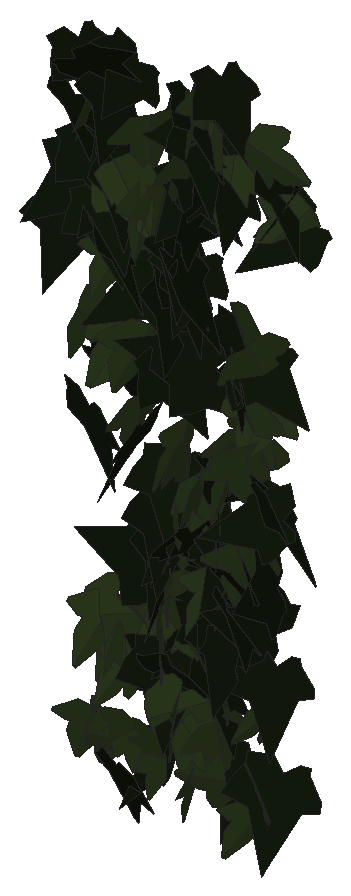
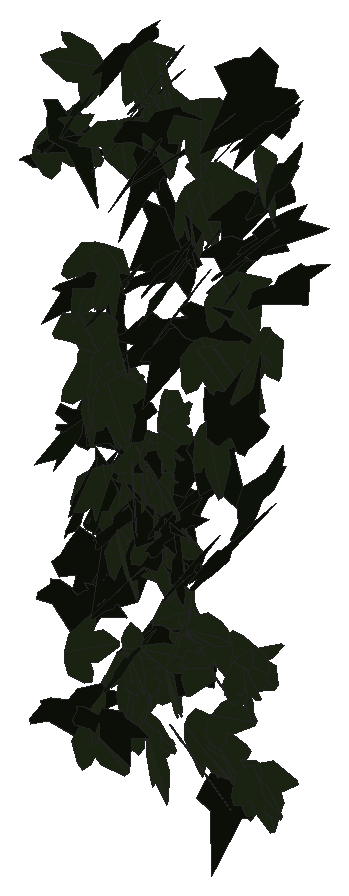
# SketchUp Ruby script. Lengths in inches.
U = 1.inch
M = Sketchup.active_model
def pt(a) = Geom::Point3d.new(a.map { |v| v * U })
def face(e, loops, mat)
  f = e.add_face(loops[0].map { |a| pt(a) })
  loops[1..].each { |l| e.add_face(l.map { |a| pt(a) }).erase! }
  f.material = f.back_material = mat if mat
  f
end
# faces: each face lists its corners as indices into pts; further lists are holes
def faces(e, pts, list, mat = nil) = list.each { |f| face(e, (f[0].is_a?(Array) ? f : [f]).map { |l| l.map { |i| pts[i] } }, mat) }
# xy, xz, yz: faces in a plane at the given z, y or x. An outline is a flat list of corners, or four numbers for a rectangle; further outlines are holes
def ring(l) = l.size == 4 ? [[l[0], l[1]], [l[2], l[1]], [l[2], l[3]], [l[0], l[3]]] : l.each_slice(2).to_a
def flat(e, list, mat, &to3) = list.each { |f| face(e, (f[0].is_a?(Array) ? f : [f]).map { |l| ring(l).map { |u, v| to3.(u, v) } }, mat) }
def xy(e, z, list, mat = nil) = flat(e, list, mat) { |x, y| [x, y, z] }
def xz(e, y, list, mat = nil) = flat(e, list, mat) { |x, z| [x, y, z] }
def yz(e, x, list, mat = nil) = flat(e, list, mat) { |y, z| [x, y, z] }
def lines(e, pts, list) = list.each { |a, b| e.add_line(pt(pts[a]), pt(pts[b])) }
# prism: a flat outline (further loops are holes) pulled along v
def prism(e, loops, v, mat = nil)
  f = face(e, loops, mat); d = Geom::Vector3d.new(v.map { |x| x * U })
  f.pushpull(f.normal.samedirection?(d) ? d.length : -d.length)
end
def box(e, o, s, mat = nil) = prism(e, [[o, [o[0] + s[0], o[1], o[2]], [o[0] + s[0], o[1] + s[1], o[2]], [o[0], o[1] + s[1], o[2]]]], [0, 0, s[2]], mat)
def at(x, y, z, deg = 0) = Geom::Transformation.translation(pt([x, y, z])) * Geom::Transformation.rotation(ORIGIN, Z_AXIS, deg.degrees)
def axes(o, x, y, z) = Geom::Transformation.new([*x, 0, *y, 0, *z, 0, *pt(o).to_a, 1])
def part(name) = M.definitions.add(name)
# library, detail: a bought-in or finely detailed component or shape, given as its bounding box
def library(name, o, s) = part(name).tap { |d| box(d.entities, o, s) }
def detail(e, o, s) = box(e.add_group.entities, o, s)
def put(e, d, t, mat = nil) = e.add_instance(d, t).tap { |i| i.material = mat if mat }
def group(e, t, mat = nil) = e.add_group.tap { |g| g.transformation = t; g.material = mat if mat }.entities
root = M.entities
M.materials.add("efeu1").color = [18, 25, 13]
M.materials.add("efeu2").color = [43, 57, 29]
c1 = part("ivyleaf_10")
p = [[0,0.5,-0.03],[-0.0625,2.02,-0.43],[-0.19,2.01,-0.46],[-0.54,1.05,-0.29],[-0.52,0.625,-0.18],[-0.83,0.76,-0.28],
  [-1.16,0.64,-0.33],[-1.15,0.33,-0.24],[-0.77,-0.39,0.02],[-0.3,-0.51,0.16],[0.04,-0.48,0.23],[-0.02,2.01,-0.4375],
  [-0.06,2.01,-0.43],[0.04,-0.49,0.23],[0.67,-0.49,0.14],[1.38,0.36,-0.2],[1.375,0.51,-0.24],[0.81,0.65,-0.19],
  [0.62,0.59,-0.15],[0.6,1.09,-0.28],[0.5,1.23,-0.31]]
faces(c1.entities,p,[[0,1,2,3,4,5,6,7,8,9,10],[11,12,0,13,14,15,16,17,18,19,20]],"efeu2")
c2 = part("ivyleaf_9")
p = [[1.54,2.16,1.25],[1.36,2.04,1.19],[-0.21,0.99,0.68],[-0.71,1.11,0.82],[-0.85,0.86,0.67],[-0.8,0.17,0.21],
  [-0.9,-0.01,0.1],[-0.67,-0.16,-0.02],[-0.08,-0.08,-0.05],[-0.03,-0.6,-0.4],[0.65,-0.88,-0.66],[0.83,-0.6,-0.49],
  [1.29,-0.42,-0.43],[1.8125,-0.07,-0.26],[1.21,0.44,0.15]]
faces(c2.entities,p,[[0,1,2,3,4,5,6,7,8,9,10,11,12,13,14]],"efeu1")
put(root,c1,axes([532.02,132.86,205.625],[0.54701,-0.58497,-0.26484],[-0.14325,0.22798,-0.79941],[0.62595,0.56337,0.04849]))
put(root,c1,axes([531.9,133,204.33],[-0.00085,-0.92422,-0.0039],[-0.00106,0.0039,-0.92422],[0.92423,-0.00084,-0.00107]))
put(root,c2,axes([532,133.3,204.76],[0.15563,-0.81555,0.1224],[0.07979,-0.10908,-0.82829],[0.82082,0.16524,0.05731]))
put(root,c2,axes([530.08,133.48,190.96],[0.09192,-0.89699,-0.19736],[0.02627,-0.1957,0.90167],[-0.91807,-0.09541,0.00604]))
put(root,c1,axes([530.97,133.13,191.32],[-0.41441,0.49964,-0.41549],[0.14606,-0.40856,-0.63699],[-0.63319,-0.42125,0.125]))
put(root,c1,axes([532.94,133.45,195],[0.0785,-0.55553,0.59073],[0.29926,-0.53176,-0.53984],[0.75368,0.269,0.15282]))
put(root,c2,axes([533.09,133.53,190.52],[0.17952,-0.61811,0.57461],[0.20391,-0.5383,-0.64274],[0.81894,0.26953,0.03408]))
put(root,c2,axes([528.87,133.62,204.78],[-0.04827,-0.74776,0.44056],[0.06981,-0.44315,-0.74452],[0.86508,-0.00596,0.08467]))
put(root,c1,axes([531.32,132.64,187.23],[0.20508,0.09961,-0.82729],[0.75248,0.3438,0.22793],[0.3579,-0.77991,-0.00518]))
put(root,c1,axes([529.61,132.87,202.91],[0.64103,0.38188,0.45288],[0.39221,0.2265,-0.74614],[-0.44397,0.75147,-0.00526]))
put(root,c2,axes([527.93,133.67,202.14],[-0.41899,-0.53929,0.51799],[-0.29131,-0.42913,-0.68241],[0.68868,-0.50962,0.02648]))
put(root,c1,axes([531.3125,133.3,187.21],[0.37585,-0.57183,0.34634],[0.24164,-0.25427,-0.68203],[0.62334,0.44336,0.05555]))
put(root,c2,axes([531.07,133.25,188.54],[-0.5829,-0.53277,-0.42244],[0.3041,0.29339,-0.78963],[0.60813,-0.65738,-0.01005]))
put(root,c2,axes([534.25,133.73,191.54],[-0.06538,-0.32194,0.83628],[-0.19736,-0.81274,-0.32831],[0.8741,-0.20758,-0.01158]))
put(root,c2,axes([531.7,133.6875,202.84],[-0.36375,-0.5854,0.46056],[0.00311,-0.51374,-0.65053],[0.74485,-0.28373,0.22764]))
put(root,c2,axes([533.47,133.58,191.86],[0.08581,-0.37368,0.77978],[0.24054,-0.74237,-0.38222],[0.83056,0.25361,0.03013]))
put(root,c2,axes([530.9375,133.47,191.24],[-0.23283,0.02472,-0.74149],[0.60895,-0.43756,-0.20579],[-0.42379,-0.64231,0.11166]))
put(root,c1,axes([530.11,133.38,202.23],[0.02057,-0.74127,0.36329],[0.24871,-0.34095,-0.70977],[0.78715,0.1271,0.21477]))
put(root,c1,axes([533.9,133.36,184.67],[-0.31046,-0.5235,0.43837],[-0.19234,-0.39501,-0.60793],[0.65515,-0.36404,0.02926]))
put(root,c2,axes([527.47,133.59,200.8125],[-0.30848,-0.78065,0.13568],[-0.03516,-0.13197,-0.83924],[0.79157,-0.31008,0.0156]))
put(root,c2,axes([531.32,133.14,200.76],[-0.21208,-0.05665,-0.91189],[0.85014,0.33069,-0.21826],[0.33469,-0.87588,-0.02342]))
put(root,c1,axes([530.51,133.07,204.72],[-0.445,-0.70945,-0.04313],[0.02158,0.03738,-0.83747],[0.71044,-0.44552,-0.00159]))
put(root,c2,axes([530.61,132.91,188.07],[0.30461,0.20191,-0.67109],[0.53531,0.40522,0.3649],[0.45229,-0.61558,0.02009]))
put(root,c2,axes([530.75,133.58,192.82],[-0.0974,-0.86981,0.11578],[-0.01013,-0.11537,-0.87524],[0.87742,-0.09789,0.00275]))
put(root,c1,axes([532.76,133.09,185.51],[-0.19611,0.02326,0.77628],[-0.77293,-0.08384,-0.19275],[0.07566,-0.79626,0.04297]))
put(root,c1,axes([532.8,133.05,187.0625],[-0.32522,-0.69186,-0.17785],[0.09706,0.1508,-0.76413],[0.70772,-0.33861,0.02307]))
put(root,c2,axes([528.99,133.6,202.4],[0.15948,-0.75012,0.28949],[0.07702,-0.27952,-0.76671],[0.80034,0.17637,0.0161]))
put(root,c2,axes([531.75,133.24,192.55],[-0.19968,0.63241,-0.49087],[0.06118,-0.49237,-0.65924],[-0.79822,-0.19594,0.07227]))
put(root,c2,axes([534.65,133.39,193.92],[-0.6743,0.00539,0.4409],[-0.44088,0.00467,-0.67432],[-0.00707,-0.80564,-0.00096]))
put(root,c2,axes([533.64,132.86,198.11],[0.13195,0.04339,-0.81934],[-0.81811,0.07003,-0.12804],[0.06236,0.82693,0.05383]))
put(root,c2,axes([532.57,132.85,190.33],[-0.16425,0.3405,0.69057],[-0.49762,0.49188,-0.36089],[-0.58755,-0.51178,0.1126]))
put(root,c2,axes([532.75,133.7,189.57],[-0.12607,-0.79959,0.20005],[0.00302,-0.20282,-0.80877],[0.82423,-0.12155,0.03356]))
put(root,c1,axes([532.54,133.59,191.13],[-0.36468,-0.56042,0.50547],[-0.09343,-0.52355,-0.64787],[0.7489,-0.33821,0.16532]))
put(root,c1,axes([530.75,132.93,185.55],[0.25194,-0.13166,-0.83357],[-0.69673,0.45841,-0.28299],[0.47618,0.74039,0.02697]))
put(root,c1,axes([531.64,133,195.34],[0.16512,-0.75649,-0.37081],[0.00109,0.37806,-0.77079],[0.84249,0.14778,0.07367]))
put(root,c2,axes([528.83,133.46,200.52],[0.44167,-0.6628,0.18007],[0.09977,-0.14991,-0.79647],[0.67954,0.4528,-0.0001]))
put(root,c1,axes([534.08,132.98,198.99],[-0.41179,-0.65559,-0.37988],[0.205,0.31983,-0.77419],[0.72944,-0.45999,0.00312]))
put(root,c2,axes([528.39,132.69,206.13],[0.73102,0.45301,0.21296],[0.16798,0.13306,-0.85968],[-0.47154,0.74969,0.0239]))
put(root,c1,axes([532.04,132.87,186.73],[0.06735,0.69163,0.36124],[0.04577,0.35846,-0.69483],[-0.77894,0.08086,-0.00959]))
put(root,c1,axes([529.9,133.52,197.82],[-0.42474,-0.67976,0.39362],[-0.15361,-0.36696,-0.79947],[0.77033,-0.44798,0.05761]))
put(root,c1,axes([534.11,133.32,205.1],[-0.23144,0.00481,-0.83159],[0.79681,-0.24578,-0.22318],[-0.23802,-0.82746,0.06145]))
put(root,c1,axes([533.61,133.3,192.45],[-0.64016,-0.52196,0.17914],[-0.13322,-0.12008,-0.82593],[0.53552,-0.65381,0.00868]))
put(root,c2,axes([532.02,133.79,197.51],[-0.31771,-0.72583,-0.52401],[-0.15763,-0.50199,0.79089],[-0.88123,0.35147,0.04745]))
put(root,c1,axes([533.76,133.18,195.65],[-0.60068,-0.74217,-0.1277],[0.08212,0.09782,-0.95479],[0.74858,-0.60627,0.00227]))
put(root,c2,axes([528.72,133.4375,201.62],[-0.17194,-0.7198,-0.35832],[0.18994,0.31969,-0.73334],[0.7813,-0.23612,0.09942]))
put(root,c1,axes([533.62,133.58,185.35],[-0.03842,-0.19654,0.74734],[0.70333,-0.31884,-0.0477],[0.3201,0.677,0.1945]))
put(root,c1,axes([528.41,133.82,188.77],[-0.34827,-0.45388,0.61207],[0.12453,-0.69782,-0.44662],[0.75175,-0.09469,0.35754]))
put(root,c1,axes([532.24,133.375,204.76],[0.76263,-0.35159,-0.01271],[-0.00688,0.01542,-0.8397],[0.35175,0.76258,0.01112]))
put(root,c2,axes([531.06,133.14,197.77],[0.15772,-0.65442,-0.58031],[-0.1554,0.55932,-0.67298],[0.86074,0.22089,-0.01517]))
put(root,c2,axes([531.06,133.5625,194.3],[-0.38912,-0.69537,-0.25303],[0.12177,0.22181,-0.79684],[0.72989,-0.40773,-0.00196]))
put(root,c1,axes([529.4,133.42,197.83],[0.82236,0.1954,-0.41509],[-0.4076,-0.07991,-0.84513],[-0.21059,0.91771,0.01479]))
put(root,c1,axes([531.02,133.78,195.02],[0.11228,-0.51871,0.57243],[0.1497,-0.55287,-0.53035],[0.75784,0.18606,0.01996]))
put(root,c2,axes([530.67,133.87,198.95],[0.07447,-0.7399,0.40506],[0.03071,-0.40398,-0.74359],[0.84296,0.08008,-0.00869]))
put(root,c2,axes([532.3,132.72,202.99],[0.13563,-0.12002,-0.95271],[-0.68535,0.66184,-0.18094],[0.67258,0.6986,0.00775]))
put(root,c2,axes([531.0625,133.93,192.04],[-0.20968,-0.564,0.47955],[-0.17641,-0.44599,-0.60167],[0.71899,-0.27391,-0.00777]))
put(root,c2,axes([532.69,133.88,203.43],[-0.00028,-0.75848,0.35794],[0.06685,-0.35682,-0.75606],[0.83603,0.02828,0.06058]))
put(root,c1,axes([533.77,133.28,196.86],[-0.75604,0.05552,-0.23432],[0.22904,-0.07256,-0.75621],[-0.07434,-0.78819,0.05311]))
put(root,c1,axes([530.57,133.6,189.42],[-0.16834,0.66822,-0.51384],[0.13799,-0.49507,-0.68902],[-0.83157,-0.21743,-0.01032]))
put(root,c2,axes([529.85,133.46,195.01],[-0.44426,0.58846,-0.47549],[0.27568,-0.38758,-0.73724],[-0.70454,-0.52272,0.01135]))
put(root,c2,axes([531.55,133.53,205.7],[0.41351,-0.7399,-0.03157],[-0.01315,0.02882,-0.8476],[0.74046,0.41371,0.00258]))
put(root,c2,axes([533.24,133.24,194.93],[0.23175,0.36283,-0.66877],[-0.56834,-0.38224,-0.40433],[-0.50585,0.59569,0.14789]))
put(root,c1,axes([528.36,132.92,198.3],[0.02079,-0.59617,-0.63833],[0.226,0.62044,-0.5721],[0.84369,-0.15151,0.16898]))
put(root,c1,axes([531.54,133.36,191.41],[-0.72603,-0.29018,0.16338],[-0.14034,-0.08877,-0.78131],[0.302,-0.73887,0.02971]))
put(root,c1,axes([532.125,133.65,205.95],[-0.06375,-0.80108,0.27625],[0.12177,-0.28281,-0.79202],[0.83858,-0.01983,0.13601]))
put(root,c1,axes([534.04,133.48,197.23],[0.81915,0.21802,-0.21675],[-0.21124,-0.049,-0.84764],[-0.22336,0.84592,0.00676]))
put(root,c1,axes([530.45,133.58,202.32],[0.0232,-0.81164,0.15371],[0.10795,-0.14947,-0.80556],[0.81898,0.0427,0.10183]))
put(root,c2,axes([533.89,133.27,198.55],[0.18121,-0.55981,-0.54317],[0.15185,0.57229,-0.53916],[0.76509,0.01901,0.23566]))
put(root,c2,axes([529.33,133.13,184.62],[0.68316,0.08931,-0.52708],[-0.52709,-0.03019,-0.68829],[-0.08921,0.86232,0.03049]))
put(root,c1,axes([529.51,133.32,185.69],[0.48392,-0.11141,-0.56654],[-0.5104,0.26307,-0.48769],[0.26996,0.69709,0.0935]))
put(root,c2,axes([532.86,133.07,193.57],[0.07781,-0.05125,-0.83119],[-0.79768,0.23516,-0.08918],[0.23916,0.80102,-0.027]))
put(root,c1,axes([528.81,133.54,188.4],[0.66233,-0.35838,-0.04558],[-0.04121,0.01961,-0.75306],[0.35891,0.6636,-0.00236]))
put(root,c2,axes([530.67,133.61,185.625],[-0.76016,0.22241,-0.20945],[0.20063,-0.06015,-0.79203],[-0.2304,-0.78619,0.00135]))
put(root,c1,axes([530.6,133.44,189.63],[0.39485,-0.03108,0.66099],[0.65552,0.12348,-0.38577],[-0.09036,0.75997,0.08971]))
put(root,c2,axes([534.34,133.87,185.74],[-0.41247,-0.80289,-0.14445],[0.06696,0.12799,-0.90264],[0.81302,-0.41787,0.00106]))
put(root,c1,axes([528.91,133.85,200.14],[-0.37708,-0.58511,0.42867],[-0.06931,-0.45186,-0.67774],[0.72202,-0.34896,0.15882]))
put(root,c2,axes([532.61,134.1,191.91],[-0.18755,-0.67235,0.37039],[-0.11821,-0.35144,-0.69781],[0.75847,-0.22103,-0.01717]))
put(root,c1,axes([534.74,134.05,202.9],[-0.34039,-0.35279,0.70404],[-0.14855,-0.72446,-0.43484],[0.77334,-0.29444,0.22636]))
put(root,c2,axes([533.9,134.02,189.93],[-0.03255,-0.02825,0.82963],[-0.68279,-0.47128,-0.04284],[0.47211,-0.68354,-0.00475]))
put(root,c2,axes([530.77,133.1875,188.59],[-0.37805,0.45583,0.49738],[-0.3044,0.39357,-0.59206],[-0.60209,-0.4852,-0.01297]))
put(root,c1,axes([531.59,133.67,185.04],[0.25174,-0.71675,0.0603],[0.01898,-0.05724,-0.75968],[0.71904,0.25245,-0.00106]))
put(root,c2,axes([532.82,134.07,198.625],[0.0468,-0.72136,0.40497],[0.11941,-0.39548,-0.71826],[0.8186,0.09893,0.08162]))
put(root,c2,axes([532.0625,134,187.98],[0.26419,-0.79338,0.35827],[0.15075,-0.32705,-0.83541],[0.85736,0.30198,0.03649]))
put(root,c2,axes([527.1875,134.02,203.99],[0.16824,-0.68104,0.48598],[0.25372,-0.43084,-0.69159],[0.79726,0.28082,0.11754]))
put(root,c2,axes([534.25,133.74,189.05],[-0.53997,-0.48823,-0.41615],[0.29295,0.29625,-0.72769],[0.57073,-0.61399,-0.0202]))
put(root,c2,axes([531.7,133.37,203.56],[0.50849,-0.54488,-0.44211],[-0.22051,0.39424,-0.73951],[0.66613,0.54644,0.09268]))
put(root,c2,axes([530.25,134.14,191.1],[-0.03594,-0.71087,0.4263],[0.00757,-0.42697,-0.71134],[0.82886,-0.02692,0.02498]))
put(root,c1,axes([533.84,134.16,187.5625],[0.01218,-0.16551,0.77293],[0.09618,-0.76697,-0.16575],[0.78458,0.09659,0.00832]))
put(root,c1,axes([532.62,133.72,191.08],[0.38821,-0.70909,0.03542],[0.0099,-0.03496,-0.80837],[0.70991,0.38825,-0.00809]))
put(root,c2,axes([532.48,133.68,206.46],[0.21299,-0.76786,-0.27667],[-0.05202,0.27259,-0.79656],[0.81453,0.21819,0.02147]))
put(root,c2,axes([532.49,133.25,191.53],[0.88769,0.19627,-0.27277],[-0.26574,-0.06161,-0.90912],[-0.20569,0.9266,-0.00267]))
put(root,c2,axes([528.19,133.64,203.3125],[0.0455,-0.81472,-0.45597],[0.00049,0.45653,-0.81568],[0.93364,0.03946,0.02265]))
put(root,c1,axes([527.88,133.75,204.29],[0.40436,-0.75752,0.05912],[0.02649,-0.05288,-0.85869],[0.75936,0.40523,-0.00153]))
put(root,c1,axes([528.9,134.14,187.22],[-0.23652,-0.29597,0.6492],[0.11012,-0.69089,-0.27485],[0.70493,0.00862,0.26076]))
put(root,c1,axes([528,133.68,185.51],[-0.61577,-0.33553,0.25023],[-0.20936,-0.13854,-0.70096],[0.36244,-0.65007,0.02023]))
put(root,c1,axes([531.41,133.32,193.14],[-0.17287,0.69239,0.3044],[-0.19944,0.25946,-0.70345],[-0.72958,-0.23499,0.12018]))
put(root,c2,axes([531.3,133.21,201.11],[-0.06232,0.12848,0.87859],[-0.43987,0.76062,-0.14243],[-0.77133,-0.44414,0.01023]))
put(root,c2,axes([534.09,133.75,194.24],[0.60191,-0.66537,-0.00201],[-0.0013,0.00154,-0.89722],[0.66537,0.60191,0.00007]))
put(root,c2,axes([534.12,134.01,203.8],[0.29613,-0.74041,0.23584],[0.11727,-0.20691,-0.79684],[0.76816,0.31702,0.03073]))
put(root,c1,axes([531.94,133.37,194.13],[0.13591,-0.68549,-0.46636],[-0.03339,0.46768,-0.69716],[0.82842,0.13131,0.04841]))
put(root,c1,axes([528.52,133.53,185.125],[-0.15938,0.05236,0.7381],[-0.73942,0.01748,-0.16091],[-0.02818,-0.75491,0.04747]))
put(root,c1,axes([532.75,133.72,203.78],[0.62588,0.55172,-0.09423],[-0.07828,-0.05367,-0.83426],[-0.55421,0.63065,0.01143]))
put(root,c1,axes([533.2,133.88,195.79],[0.02519,-0.77462,0.1506],[-0.01404,-0.15109,-0.77481],[0.789,0.02204,-0.01859]))
put(root,c1,axes([532.76,133.28,187.63],[0.17921,-0.14057,-0.81291],[-0.51976,0.62677,-0.22297],[0.64065,0.54781,0.04651]))
put(root,c1,axes([532.89,133.86,195.59],[-0.14946,-0.75542,0.15525],[-0.01017,-0.1562,-0.7698],[0.77114,-0.14847,0.01994]))
put(root,c2,axes([531.43,134.09,204.63],[-0.43645,-0.74024,-0.11235],[0.05193,0.09981,-0.85931],[0.74692,-0.43949,-0.00591]))
put(root,c1,axes([528.34,133.63,188.79],[0.24505,-0.08512,-0.88949],[0.89094,-0.04729,0.24997],[-0.06836,-0.92142,0.06934]))
put(root,c2,axes([534.88,134.3,202.625],[-0.57951,-0.41741,0.38754],[-0.22401,-0.34129,-0.70256],[0.52368,-0.6079,0.12833]))
put(root,c1,axes([531.87,133.6,193.97],[-0.38654,-0.61967,-0.34452],[0.32702,0.19234,-0.71286],[0.62908,-0.48074,0.15888]))
put(root,c2,axes([533.18,134.01,185.71],[-0.6546,-0.35747,-0.23831],[0.20488,0.12202,-0.7458],[0.37763,-0.68586,-0.00847]))
put(root,c2,axes([530.82,134.125,199.71],[0.27974,-0.74988,0.2179],[0.07008,-0.20642,-0.80033],[0.77775,0.28831,-0.00626]))
put(root,c2,axes([528.71,133.95,196],[0.661,-0.36637,0.42115],[-0.33495,0.26185,0.7535],[-0.44654,-0.73873,0.05822]))
put(root,c2,axes([528.9375,134.42,205.45],[-0.26918,-0.64368,0.49469],[0.05855,-0.53521,-0.66454],[0.8097,-0.17528,0.21251]))
put(root,c1,axes([529.52,133.84,195.5],[-0.02186,-0.84255,0.00958],[0.00046,-0.00959,-0.84284],[0.84261,-0.02186,0.00071]))
put(root,c2,axes([531.17,134.29,200.27],[-0.2419,-0.76392,0.18614],[0.01378,-0.19884,-0.79813],[0.78616,-0.23157,0.07127]))
put(root,c2,axes([527.5,134.23,194.47],[0.36613,-0.76582,0.44652],[0.19953,-0.39952,-0.84881],[0.86374,0.41691,0.00681]))
put(root,c2,axes([527.48,133.84,205.88],[0.25665,-0.75527,-0.28664],[0.01676,0.30567,-0.79041],[0.80766,0.23366,0.10749]))
put(root,c2,axes([528.28,134.42,201.57],[-0.28876,-0.61238,0.45857],[-0.0053,-0.48854,-0.65573],[0.76503,-0.23452,0.16855]))
put(root,c1,axes([533.17,133.37,195.8],[-0.03637,-0.51541,-0.59691],[0.14142,0.5836,-0.51253],[0.77585,-0.13054,0.06544]))
put(root,c2,axes([532.34,133.55,192.34],[-0.32502,0.35882,0.61035],[-0.50709,0.35071,-0.47621],[-0.4941,-0.59596,0.08724]))
put(root,c1,axes([532.96,133.87,199.34],[-0.59473,0.41409,-0.37892],[0.26608,-0.2781,-0.72153],[-0.49422,-0.64803,0.06751]))
put(root,c1,axes([530.99,133.9,192.875],[0.60838,-0.315,-0.53264],[0.49033,-0.21029,0.68441],[-0.37751,-0.78078,0.03055]))
put(root,c1,axes([529.43,133.77,189.41],[-0.61257,0.1189,-0.4308],[0.42312,-0.08099,-0.624],[-0.14386,-0.74449,-0.00092]))
put(root,c2,axes([534.65,133.53,203.36],[-0.39834,0.77075,0.07487],[-0.03178,0.06785,-0.8676],[-0.77373,-0.3996,-0.00291]))
put(root,c2,axes([530.56,134.31,200.68],[0.07253,-0.82185,0.23649],[0.01381,-0.23619,-0.82502],[0.85509,0.07352,-0.00674]))
put(root,c2,axes([529.92,134.2,199.17],[-0.71583,-0.23108,0.31821],[-0.30309,-0.09693,-0.7522],[0.25059,-0.77735,-0.0008]))
put(root,c1,axes([530.06,133.78,188.42],[-0.05662,-0.14446,-0.8194],[0.8306,-0.05798,-0.04717],[-0.0488,-0.8193,0.14782]))
